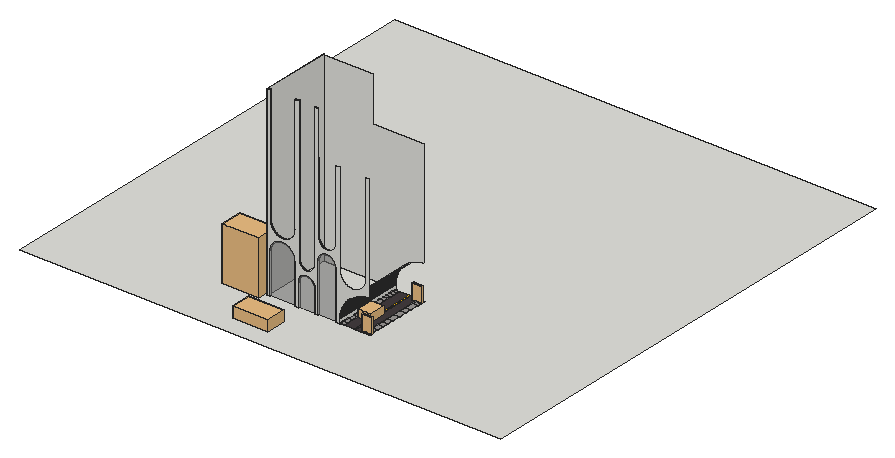
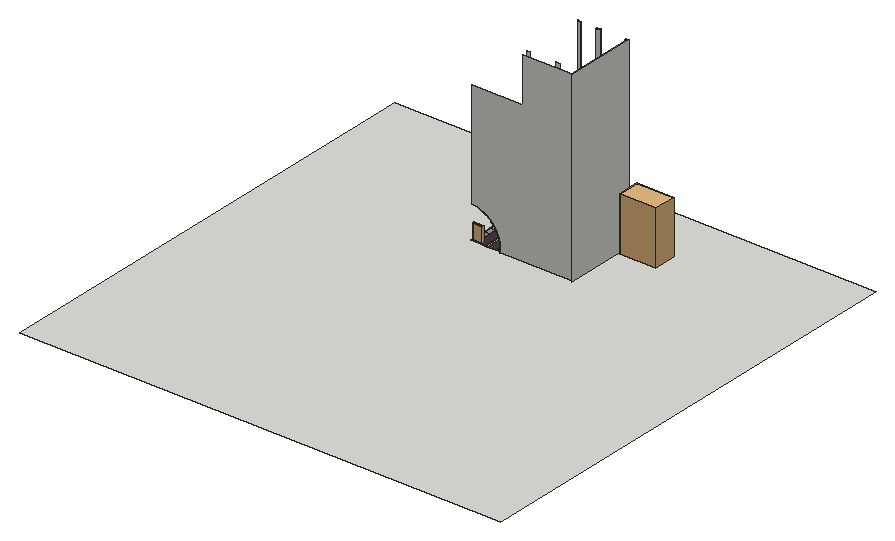
# SketchUp Ruby script. Lengths in inches.
U = 1.inch
M = Sketchup.active_model
def pt(a) = Geom::Point3d.new(a.map { |v| v * U })
def face(e, loops, mat)
  f = e.add_face(loops[0].map { |a| pt(a) })
  loops[1..].each { |l| e.add_face(l.map { |a| pt(a) }).erase! }
  f.material = f.back_material = mat if mat
  f
end
# faces: each face lists its corners as indices into pts; further lists are holes
def faces(e, pts, list, mat = nil) = list.each { |f| face(e, (f[0].is_a?(Array) ? f : [f]).map { |l| l.map { |i| pts[i] } }, mat) }
# xy, xz, yz: faces in a plane at the given z, y or x. An outline is a flat list of corners, or four numbers for a rectangle; further outlines are holes
def ring(l) = l.size == 4 ? [[l[0], l[1]], [l[2], l[1]], [l[2], l[3]], [l[0], l[3]]] : l.each_slice(2).to_a
def flat(e, list, mat, &to3) = list.each { |f| face(e, (f[0].is_a?(Array) ? f : [f]).map { |l| ring(l).map { |u, v| to3.(u, v) } }, mat) }
def xy(e, z, list, mat = nil) = flat(e, list, mat) { |x, y| [x, y, z] }
def xz(e, y, list, mat = nil) = flat(e, list, mat) { |x, z| [x, y, z] }
def yz(e, x, list, mat = nil) = flat(e, list, mat) { |y, z| [x, y, z] }
def lines(e, pts, list) = list.each { |a, b| e.add_line(pt(pts[a]), pt(pts[b])) }
# prism: a flat outline (further loops are holes) pulled along v
def prism(e, loops, v, mat = nil)
  f = face(e, loops, mat); d = Geom::Vector3d.new(v.map { |x| x * U })
  f.pushpull(f.normal.samedirection?(d) ? d.length : -d.length)
end
def box(e, o, s, mat = nil) = prism(e, [[o, [o[0] + s[0], o[1], o[2]], [o[0] + s[0], o[1] + s[1], o[2]], [o[0], o[1] + s[1], o[2]]]], [0, 0, s[2]], mat)
def at(x, y, z, deg = 0) = Geom::Transformation.translation(pt([x, y, z])) * Geom::Transformation.rotation(ORIGIN, Z_AXIS, deg.degrees)
def axes(o, x, y, z) = Geom::Transformation.new([*x, 0, *y, 0, *z, 0, *pt(o).to_a, 1])
def part(name) = M.definitions.add(name)
# library, detail: a bought-in or finely detailed component or shape, given as its bounding box
def library(name, o, s) = part(name).tap { |d| box(d.entities, o, s) }
def detail(e, o, s) = box(e.add_group.entities, o, s)
def put(e, d, t, mat = nil) = e.add_instance(d, t).tap { |i| i.material = mat if mat }
def group(e, t, mat = nil) = e.add_group.tap { |g| g.transformation = t; g.material = mat if mat }.entities
root = M.entities
M.materials.add("Asphalt_New").color = [67, 60, 62]
M.materials.add("Color_D01").color = [255, 191, 0]
M.materials.add("Concrete_Aggregate_Smoke").color = [154, 150, 148]
M.materials.add("[Translucent Glass Gray]").color = [128, 128, 128]
M.materials["[Translucent Glass Gray]"].alpha = 0.5
c1 = library("ske72",[-9.6875,-115.78,0],[19.375,125.47,218.23])
c2 = part("road")
xy(c2.entities,0,[[0,61.25,879,180.3125],[0,193.18,879,202.26],[0,211.38,879,312.5]],"Asphalt_New")
xy(c2.entities,0,[[0,180.3125,879,193.18],[0,202.26,879,211.38]],"Color_D01")
xy(c2.entities,2.25,[[0,0,58.96,61.25],[58.96,0,130.63,61.25],[130.63,0,205.31,61.25],[205.31,0,271.13,61.25],[271.13,0,347.96,61.25],
  [347.96,0,422.25,61.25],[422.25,0,490,61.25],[490,0,565.64,61.25],[565.64,0,642.8125,61.25],[642.8125,0,697.3125,61.25],
  [697.3125,0,742.61,61.25],[742.61,0,787.91,61.25],[787.91,0,833.2,61.25],[833.2,0,878.5,61.25],[0,312.5,55.73,383],
  [55.73,312.5,137.52,383],[137.52,312.5,221.8,383],[221.8,312.5,297.83,383],[297.83,312.5,375.9,383],[375.9,312.5,479.79,383],
  [479.79,312.5,571.31,383],[571.31,312.5,662.56,383],[662.56,312.5,768.4,383],[768.4,312.5,821.33,383],[821.33,312.5,874.25,383]],"Concrete_Aggregate_Smoke")
xz(c2.entities,0,[[0,0,58.96,2.25],[58.96,0,130.63,2.25],[130.63,0,205.31,2.25],[205.31,0,271.13,2.25],[271.13,0,347.96,2.25],
  [347.96,0,422.25,2.25],[422.25,0,490,2.25],[490,0,565.64,2.25],[565.64,0,604.23,2.25],[604.23,0,642.8125,2.25],
  [642.8125,0,697.3125,2.25],[697.3125,0,742.61,2.25],[742.61,0,787.91,2.25],[787.91,0,833.2,2.25],[833.2,0,878.5,2.25]],"Concrete_Aggregate_Smoke")
xz(c2.entities,61.25,[[0,0,58.96,2.25],[58.96,0,130.63,2.25],[130.63,0,205.31,2.25],[205.31,0,271.13,2.25],[271.13,0,347.96,2.25],
  [347.96,0,422.25,2.25],[422.25,0,490,2.25],[490,0,565.64,2.25],[565.64,0,642.8125,2.25],[642.8125,0,697.3125,2.25],
  [697.3125,0,742.61,2.25],[742.61,0,787.91,2.25],[787.91,0,833.2,2.25],[833.2,0,878.5,2.25]],"Concrete_Aggregate_Smoke")
xz(c2.entities,312.5,[[0,0,55.73,2.25],[55.73,0,137.52,2.25],[137.52,0,221.8,2.25],[221.8,0,297.83,2.25],[297.83,0,373.56,2.25],
  [373.56,0,375.9,2.25],[375.9,0,479.79,2.25],[479.79,0,571.31,2.25],[571.31,0,662.56,2.25],[662.56,0,768.4,2.25],
  [768.4,0,821.33,2.25],[821.33,0,874.25,2.25]],"Concrete_Aggregate_Smoke")
xz(c2.entities,383,[[0,0,55.73,2.25],[55.73,0,137.52,2.25],[137.52,0,221.8,2.25],[221.8,0,297.83,2.25],[297.83,0,375.9,2.25],
  [375.9,0,479.79,2.25],[479.79,0,571.31,2.25],[571.31,0,662.56,2.25],[662.56,0,768.4,2.25],[768.4,0,821.33,2.25],
  [821.33,0,874.25,2.25]],"Concrete_Aggregate_Smoke")
yz(c2.entities,0,[[0,0,61.25,2.25],[312.5,0,383,2.25]],"Concrete_Aggregate_Smoke")
yz(c2.entities,874.25,[[312.5,0,383,2.25]],"Concrete_Aggregate_Smoke")
yz(c2.entities,878.5,[[0,0,61.25,2.25]],"Concrete_Aggregate_Smoke")
p = [[0,0,0],[-0.25,0,0]]
lines(c2.entities,p,[[0,1]])
put(c2.entities,c1,at(36.91,376.45,-15.96))
put(c2.entities,c1,at(842.66,376.45,-15.96))
c3 = library("2016+Honda+Civic+LX+Sedan",[0.01,0.03,0.02],[16.17,34.46,10.62])
c4 = library("006_cordyline_australis",[-46.19,-61.57,-0.26],[141.35,155.27,163.93])
c5 = library("car",[-0.875,0,0],[16.18,34.45,10.62])
xy(root,0,[[0,0,3621,3534]])
xz(root,487.08,[[1470.625,0,1494.625,0,1494.625,300.79,1494.8125,306.78,1495.375,312.74,1496.3125,318.66,1497.62,324.51,1499.29,330.27,1501.32,335.9,1503.7,341.4,1506.42,346.74,1509.47,351.9,1512.84,356.86,1516.52,361.59,1520.48,366.09,1524.72,370.33,1529.21,374.29,1533.95,377.96,1538.9,381.33,1544.0625,384.38,1549.4,387.1,1554.9,389.48,1560.54,391.51,1566.3,393.1875,1572.14,394.49,1578.0625,395.43,1584.03,395.99,1590.02,396.18,1596.01,395.99,1601.98,395.43,1607.9,394.49,1613.74,393.1875,1619.5,391.51,1625.14,389.48,1630.64,387.1,1635.98,384.38,1641.14,381.33,1646.09,377.96,1650.83,374.29,1655.32,370.33,1659.5625,366.09,1663.52,361.59,1667.2,356.86,1670.57,351.9,1673.62,346.74,1676.34,341.4,1678.72,335.9,1680.75,330.27,1682.42,324.51,1683.73,318.66,1684.66,312.74,1685.23,306.78,1685.42,300.79,1685.42,0,1709.42,0,1709.42,171.3125,1709.54,175.19,1709.9,179.04,1710.51,182.87,1711.35,186.65,1712.43,190.37,1713.75,194.01,1715.28,197.5625,1717.04,201.01,1719.01,204.35,1721.19,207.55,1723.5625,210.61,1726.125,213.52,1728.86,216.26,1731.77,218.82,1734.83,221.19,1738.03,223.37,1741.37,225.34,1744.82,227.1,1748.37,228.63,1752.02,229.95,1755.73,231.03,1759.51,231.87,1763.34,232.48,1767.2,232.84,1771.07,232.96,1774.9375,232.84,1778.79,232.48,1782.62,231.87,1786.4,231.03,1790.12,229.95,1793.76,228.63,1797.32,227.1,1800.77,225.34,1804.1,223.37,1807.3,221.19,1810.36,218.82,1813.27,216.26,1816.01,213.52,1818.57,210.61,1820.94,207.55,1823.12,204.35,1825.09,201.01,1826.85,197.5625,1828.39,194.01,1829.7,190.37,1830.78,186.65,1831.625,182.87,1832.23,179.04,1832.59,175.19,1832.72,171.3125,1832.72,0,1856.72,0,1856.72,362.73,1856.85,366.99,1857.25,371.24,1857.92,375.46,1858.85,379.62,1860.04,383.72,1861.49,387.74,1863.18,391.65,1865.12,395.45,1867.29,399.13,1869.6875,402.66,1872.3,406.03,1875.125,409.23,1878.14,412.25,1881.35,415.07,1884.72,417.68,1888.25,420.08,1891.92,422.26,1895.72,424.19,1899.64,425.89,1903.65,427.33,1907.75,428.52,1911.92,429.45,1916.13,430.12,1920.38,430.52,1924.64,430.66,1928.91,430.52,1933.16,430.12,1937.37,429.45,1941.54,428.52,1945.64,427.33,1949.65,425.89,1953.57,424.19,1957.125,422.38,1957.37,422.26,1961.04,420.08,1964.57,417.68,1967.94,415.07,1971.14,412.25,1974.16,409.23,1976.98,406.03,1979.6,402.66,1982,399.13,1984.17,395.45,1986.11,391.65,1987.8,387.74,1989.25,383.72,1990.4375,379.62,1991.37,375.46,1992.04,371.24,1992.4375,366.99,1992.57,362.73,1992.57,0,2019.16,0,2018.78,7.52,2018.64,15.05,2018.74,22.58,2019.07,30.1,2019.16,31.18,2019.64,37.6,2020.44,45.09,2021.48,52.55,2022.75,59.97,2024.25,67.35,2025.98,74.67,2027.94,81.94,2030.13,89.15,2032.54,96.28,2035.17,103.33,2038.02,110.3,2041.09,117.18,2044.375,123.95,2047.87,130.62,2051.57,137.18,2055.47,143.62,2059.57,149.93,2063.875,156.11,2068.36,162.15,2073.04,168.05,2077.9,173.8,2082.94,179.4,2088.14,184.84,2093.52,190.11,2099.06,195.21,2104.76,200.13,2110.6,204.87,2116.6,209.43,2122.73,213.8,2129,217.97,2135.39,221.95,2141.9,225.72,2148.53,229.29,2155.27,232.64,2162.11,235.79,2169.05,238.72,2176.07,241.43,2183.18,243.92,2190.36,246.19,2197.6,248.23,2204.91,250.04,2212.27,251.63,2218.1,252.69,2219.68,252.98,2227.12,254.1,2233.1,254.8125,2234.6,254.99,2242.1,255.64,2242.1,1054,2218.1,1054,2218.1,364.18,2217.9,357.93,2217.3125,351.71,2216.34,345.54,2214.97,339.4375,2213.23,333.4375,2211.11,327.56,2208.63,321.82,2205.79,316.26,2202.61,310.88,2199.1,305.71,2195.27,300.77,2191.14,296.08,2186.72,291.67,2182.03,287.53,2177.09,283.7,2171.93,280.19,2166.55,277.01,2160.98,274.17,2155.24,271.69,2149.37,269.57,2143.36,267.83,2137.27,266.47,2131.09,265.49,2124.87,264.9,2118.63,264.71,2112.38,264.9,2106.16,265.49,2099.99,266.47,2093.89,267.83,2087.89,269.57,2082.01,271.69,2076.27,274.17,2070.71,277.01,2065.33,280.19,2060.16,283.7,2055.22,287.53,2050.53,291.67,2046.12,296.08,2041.98,300.77,2038.15,305.71,2034.64,310.88,2031.46,316.26,2028.62,321.82,2026.14,327.56,2024.02,333.4375,2022.28,339.4375,2020.92,345.54,2019.94,351.71,2019.35,357.93,2019.16,364.18,2019.16,1054,1992.57,1054,1992.57,527,1992.4375,522.73,1992.04,518.49,1991.37,514.27,1990.4375,510.11,1989.25,506.01,1987.8,501.99,1986.11,498.08,1984.17,494.28,1982,490.6,1979.6,487.07,1976.98,483.7,1974.16,480.5,1971.14,477.48,1967.94,474.66,1964.57,472.04,1961.04,469.65,1957.37,467.47,1953.57,465.54,1949.65,463.84,1945.64,462.4,1941.54,461.21,1937.37,460.27,1933.16,459.61,1928.91,459.21,1924.64,459.07,1920.38,459.21,1916.13,459.61,1911.92,460.27,1907.75,461.21,1903.65,462.4,1899.64,463.84,1895.72,465.54,1891.92,467.47,1888.25,469.65,1884.72,472.04,1881.35,474.66,1878.14,477.48,1875.125,480.5,1872.3,483.7,1869.6875,487.07,1867.29,490.6,1865.12,494.28,1863.18,498.08,1861.49,501.99,1860.04,506.01,1858.85,510.11,1857.92,514.27,1857.25,518.49,1856.85,522.73,1856.72,527,1856.72,1394,1832.72,1394,1832.72,325.5,1832.59,321.63,1832.23,317.77,1831.625,313.95,1830.78,310.17,1829.7,306.45,1828.39,302.8,1826.85,299.25,1825.09,295.8,1823.12,292.47,1820.94,289.26,1818.57,286.2,1816.01,283.3,1813.27,280.56,1810.36,278,1807.3,275.625,1804.1,273.45,1800.77,271.48,1797.32,269.72,1793.76,268.18,1790.12,266.87,1786.4,265.79,1782.62,264.94,1778.79,264.34,1774.9375,263.97,1771.07,263.85,1767.2,263.97,1763.34,264.34,1759.51,264.94,1755.73,265.79,1752.02,266.87,1748.37,268.18,1744.82,269.72,1741.37,271.48,1738.03,273.45,1734.83,275.625,1731.77,278,1728.86,280.56,1726.125,283.3,1723.5625,286.2,1721.19,289.26,1719.01,292.47,1717.04,295.8,1715.28,299.25,1713.75,302.8,1712.43,306.45,1711.35,310.17,1710.51,313.95,1709.9,317.77,1709.54,321.63,1709.42,325.5,1709.42,1394,1685.42,1394,1685.42,523.51,1685.82,517.14,1685.79,510.75,1685.42,505.5,1685.34,504.38,1684.46,498.05,1683.17,491.8,1681.46,485.64,1679.34,479.62,1676.83,473.74,1673.93,468.05,1670.66,462.5625,1667.03,457.31,1663.0625,452.3,1658.77,447.57,1654.17,443.14,1649.28,439.03,1644.13,435.25,1638.74,431.82,1633.14,428.76,1627.34,426.07,1621.375,423.78,1615.27,421.9,1609.06,420.42,1602.76,419.36,1596.4,418.72,1590.02,418.51,1583.64,418.72,1577.28,419.36,1570.98,420.42,1564.77,421.9,1558.66,423.78,1552.7,426.07,1546.9,428.76,1541.3,431.82,1535.91,435.25,1530.76,439.03,1525.875,443.14,1521.27,447.57,1516.98,452.3,1513.01,457.31,1509.38,462.5625,1506.11,468.05,1503.21,473.74,1500.7,479.62,1498.58,485.64,1496.875,491.8,1495.58,498.05,1494.7,504.38,1494.625,505.5,1494.25,510.75,1494.22,517.14,1494.625,523.51,1494.625,1394,1470.625,1394],[2019.16,0,2019.16,31.18,2019.07,30.1,2018.74,22.58,2018.64,15.05,2018.78,7.52]])
xz(root,487.08,[[1494.625,0,1685.42,0,1685.42,300.79,1685.23,306.78,1684.66,312.74,1683.73,318.66,1682.42,324.51,1680.75,330.27,1678.72,335.9,1676.34,341.4,1673.62,346.74,1670.57,351.9,1667.2,356.86,1663.52,361.59,1659.5625,366.09,1655.32,370.33,1650.83,374.29,1646.09,377.96,1641.14,381.33,1635.98,384.38,1630.64,387.1,1625.14,389.48,1619.5,391.51,1613.74,393.1875,1607.9,394.49,1601.98,395.43,1596.01,395.99,1590.02,396.18,1584.03,395.99,1578.0625,395.43,1572.14,394.49,1566.3,393.1875,1560.54,391.51,1554.9,389.48,1549.4,387.1,1544.0625,384.38,1538.9,381.33,1533.95,377.96,1529.21,374.29,1524.72,370.33,1520.48,366.09,1516.52,361.59,1512.84,356.86,1509.47,351.9,1506.42,346.74,1503.7,341.4,1501.32,335.9,1499.29,330.27,1497.62,324.51,1496.3125,318.66,1495.375,312.74,1494.8125,306.78,1494.625,300.79],[1709.42,0,1832.72,0,1832.72,171.3125,1832.59,175.19,1832.23,179.04,1831.625,182.87,1830.78,186.65,1829.7,190.37,1828.39,194.01,1826.85,197.5625,1825.09,201.01,1823.12,204.35,1820.94,207.55,1818.57,210.61,1816.01,213.52,1813.27,216.26,1810.36,218.82,1807.3,221.19,1804.1,223.37,1800.77,225.34,1797.32,227.1,1793.76,228.63,1790.12,229.95,1786.4,231.03,1782.62,231.87,1778.79,232.48,1774.9375,232.84,1771.07,232.96,1767.2,232.84,1763.34,232.48,1759.51,231.87,1755.73,231.03,1752.02,229.95,1748.37,228.63,1744.82,227.1,1741.37,225.34,1738.03,223.37,1734.83,221.19,1731.77,218.82,1728.86,216.26,1726.125,213.52,1723.5625,210.61,1721.19,207.55,1719.01,204.35,1717.04,201.01,1715.28,197.5625,1713.75,194.01,1712.43,190.37,1711.35,186.65,1710.51,182.87,1709.9,179.04,1709.54,175.19,1709.42,171.3125],[1856.72,0,1992.57,0,1992.57,362.73,1992.4375,366.99,1992.04,371.24,1991.37,375.46,1990.4375,379.62,1989.25,383.72,1987.8,387.74,1986.11,391.65,1984.17,395.45,1982,399.13,1979.6,402.66,1976.98,406.03,1974.16,409.23,1971.14,412.25,1967.94,415.07,1964.57,417.68,1961.04,420.08,1957.37,422.26,1953.57,424.19,1949.65,425.89,1945.64,427.33,1941.54,428.52,1937.37,429.45,1933.16,430.12,1928.91,430.52,1924.64,430.66,1920.38,430.52,1916.13,430.12,1911.92,429.45,1907.75,428.52,1903.65,427.33,1899.64,425.89,1895.72,424.19,1891.92,422.26,1888.25,420.08,1884.72,417.68,1881.35,415.07,1878.14,412.25,1875.125,409.23,1872.3,406.03,1869.6875,402.66,1867.29,399.13,1865.12,395.45,1863.18,391.65,1861.49,387.74,1860.04,383.72,1858.85,379.62,1857.92,375.46,1857.25,371.24,1856.85,366.99,1856.72,362.73]],"[Translucent Glass Gray]")
xz(root,496.08,[[1479.625,0,1479.625,1394,1494.625,1394,1494.625,505.5,1494.7,504.38,1495.58,498.05,1496.875,491.8,1498.58,485.64,1500.7,479.62,1503.21,473.74,1506.11,468.05,1509.38,462.5625,1513.01,457.31,1516.98,452.3,1521.27,447.57,1525.875,443.14,1530.76,439.03,1535.91,435.25,1541.3,431.82,1546.9,428.76,1552.7,426.07,1558.66,423.78,1564.77,421.9,1570.98,420.42,1577.28,419.36,1583.64,418.72,1590.02,418.51,1596.4,418.72,1602.76,419.36,1609.06,420.42,1615.27,421.9,1621.375,423.78,1627.34,426.07,1633.14,428.76,1638.74,431.82,1644.13,435.25,1649.28,439.03,1654.17,443.14,1658.77,447.57,1663.0625,452.3,1667.03,457.31,1670.66,462.5625,1673.93,468.05,1676.83,473.74,1679.34,479.62,1681.46,485.64,1683.17,491.8,1684.46,498.05,1685.34,504.38,1685.42,505.5,1685.42,1394,1709.42,1394,1709.42,325.5,1709.54,321.63,1709.9,317.77,1710.51,313.95,1711.35,310.17,1712.43,306.45,1713.75,302.8,1715.28,299.25,1717.04,295.8,1719.01,292.47,1721.19,289.26,1723.5625,286.2,1726.125,283.3,1728.86,280.56,1731.77,278,1734.83,275.625,1738.03,273.45,1741.37,271.48,1744.82,269.72,1748.37,268.18,1752.02,266.87,1755.73,265.79,1759.51,264.94,1763.34,264.34,1767.2,263.97,1771.07,263.85,1774.9375,263.97,1778.79,264.34,1782.62,264.94,1786.4,265.79,1790.12,266.87,1793.76,268.18,1797.32,269.72,1800.77,271.48,1804.1,273.45,1807.3,275.625,1810.36,278,1813.27,280.56,1816.01,283.3,1818.57,286.2,1820.94,289.26,1823.12,292.47,1825.09,295.8,1826.85,299.25,1828.39,302.8,1829.7,306.45,1830.78,310.17,1831.625,313.95,1832.23,317.77,1832.59,321.63,1832.72,325.5,1832.72,1394,1847.72,1394,1847.72,1054,1856.72,1054,1856.72,527,1856.85,522.73,1857.25,518.49,1857.92,514.27,1858.85,510.11,1860.04,506.01,1861.49,501.99,1863.18,498.08,1865.12,494.28,1867.29,490.6,1869.6875,487.07,1872.3,483.7,1875.125,480.5,1878.14,477.48,1881.35,474.66,1884.72,472.04,1888.25,469.65,1891.92,467.47,1895.72,465.54,1899.64,463.84,1903.65,462.4,1907.75,461.21,1911.92,460.27,1916.13,459.61,1920.38,459.21,1924.64,459.07,1928.91,459.21,1933.16,459.61,1937.37,460.27,1941.54,461.21,1945.64,462.4,1949.65,463.84,1953.57,465.54,1957.125,467.35,1957.125,422.38,1953.57,424.19,1949.65,425.89,1945.64,427.33,1941.54,428.52,1937.37,429.45,1933.16,430.12,1928.91,430.52,1924.64,430.66,1920.38,430.52,1916.13,430.12,1911.92,429.45,1907.75,428.52,1903.65,427.33,1899.64,425.89,1895.72,424.19,1891.92,422.26,1888.25,420.08,1884.72,417.68,1881.35,415.07,1878.14,412.25,1875.125,409.23,1872.3,406.03,1869.6875,402.66,1867.29,399.13,1865.12,395.45,1863.18,391.65,1861.49,387.74,1860.04,383.72,1858.85,379.62,1857.92,375.46,1857.25,371.24,1856.85,366.99,1856.72,362.73,1856.72,0,1832.72,0,1832.72,171.3125,1832.59,175.19,1832.23,179.04,1831.625,182.87,1830.78,186.65,1829.7,190.37,1828.39,194.01,1826.85,197.5625,1825.09,201.01,1823.12,204.35,1820.94,207.55,1818.57,210.61,1816.01,213.52,1813.27,216.26,1810.36,218.82,1807.3,221.19,1804.1,223.37,1800.77,225.34,1797.32,227.1,1793.76,228.63,1790.12,229.95,1786.4,231.03,1782.62,231.87,1778.79,232.48,1774.9375,232.84,1771.07,232.96,1767.2,232.84,1763.34,232.48,1759.51,231.87,1755.73,231.03,1752.02,229.95,1748.37,228.63,1744.82,227.1,1741.37,225.34,1738.03,223.37,1734.83,221.19,1731.77,218.82,1728.86,216.26,1726.125,213.52,1723.5625,210.61,1721.19,207.55,1719.01,204.35,1717.04,201.01,1715.28,197.5625,1713.75,194.01,1712.43,190.37,1711.35,186.65,1710.51,182.87,1709.9,179.04,1709.54,175.19,1709.42,171.3125,1709.42,0,1685.42,0,1685.42,300.79,1685.23,306.78,1684.66,312.74,1683.73,318.66,1682.42,324.51,1680.75,330.27,1678.72,335.9,1676.34,341.4,1673.62,346.74,1670.57,351.9,1667.2,356.86,1663.52,361.59,1659.5625,366.09,1655.32,370.33,1650.83,374.29,1646.09,377.96,1641.14,381.33,1635.98,384.38,1630.64,387.1,1625.14,389.48,1619.5,391.51,1613.74,393.1875,1607.9,394.49,1601.98,395.43,1596.01,395.99,1590.02,396.18,1584.03,395.99,1578.0625,395.43,1572.14,394.49,1566.3,393.1875,1560.54,391.51,1554.9,389.48,1549.4,387.1,1544.0625,384.38,1538.9,381.33,1533.95,377.96,1529.21,374.29,1524.72,370.33,1520.48,366.09,1516.52,361.59,1512.84,356.86,1509.47,351.9,1506.42,346.74,1503.7,341.4,1501.32,335.9,1499.29,330.27,1497.62,324.51,1496.3125,318.66,1495.375,312.74,1494.8125,306.78,1494.625,300.79,1494.625,0]])
xz(root,1012.08,[[1479.625,0,2019.16,0,2019.16,31.18,2019.64,37.6,2020.44,45.09,2021.48,52.55,2022.75,59.97,2024.25,67.35,2025.98,74.67,2027.94,81.94,2030.13,89.15,2032.54,96.28,2035.17,103.33,2038.02,110.3,2041.09,117.18,2044.375,123.95,2047.87,130.62,2051.57,137.18,2055.47,143.62,2059.57,149.93,2063.875,156.11,2068.36,162.15,2073.04,168.05,2077.9,173.8,2082.94,179.4,2088.14,184.84,2093.52,190.11,2099.06,195.21,2104.76,200.13,2110.6,204.87,2116.6,209.43,2122.73,213.8,2129,217.97,2135.39,221.95,2141.9,225.72,2148.53,229.29,2155.27,232.64,2162.11,235.79,2169.05,238.72,2176.07,241.43,2183.18,243.92,2190.36,246.19,2197.6,248.23,2204.91,250.04,2212.27,251.63,2218.1,252.69,2219.68,252.98,2227.12,254.1,2233.1,254.8125,2233.1,1054,1847.72,1054,1847.72,1394,1479.625,1394]])
yz(root,1470.625,[[487.08,0,1021.08,1394]])
yz(root,1479.625,[[496.08,0,1012.08,1394]])
yz(root,1494.625,[[487.08,0,496.08,300.79]])
yz(root,1685.42,[[487.08,0,496.08,300.79]])
yz(root,1709.42,[[487.08,0,496.08,171.3125]])
yz(root,1832.72,[[487.08,0,496.08,171.3125]])
yz(root,1856.72,[[487.08,0,496.08,362.73]])
yz(root,1992.57,[[487.08,0,496.08,362.73]])
yz(root,2019.16,[[487.08,0,1012.08,31.18]])
p = [[2019.64,487.08,37.6],[2019.16,487.08,31.18],[2019.16,1012.08,31.18],[2019.64,1012.08,37.6],[2020.44,1012.08,45.09],[2020.44,487.08,45.09],
  [2021.48,487.08,52.55],[2021.48,1012.08,52.55],[2022.75,487.08,59.97],[2022.75,1012.08,59.97],[2024.25,487.08,67.35],[2024.25,1012.08,67.35],
  [2025.98,487.08,74.67],[2025.98,1012.08,74.67],[2027.94,487.08,81.94],[2027.94,1012.08,81.94],[2030.13,487.08,89.15],[2030.13,1012.08,89.15],
  [2032.54,1012.08,96.28],[2032.54,487.08,96.28],[2035.17,487.08,103.33],[2035.17,1012.08,103.33],[2038.02,487.08,110.3],[2038.02,1012.08,110.3],
  [2041.09,487.08,117.18],[2041.09,1012.08,117.18],[2044.375,487.08,123.95],[2044.375,1012.08,123.95],[2047.87,487.08,130.62],[2047.87,1012.08,130.62],
  [2051.57,487.08,137.18],[2051.57,1012.08,137.18],[2055.47,487.08,143.62],[2055.47,1012.08,143.62],[2059.57,487.08,149.93],[2059.57,1012.08,149.93],
  [2063.875,487.08,156.11],[2063.875,1012.08,156.11],[2068.36,487.08,162.15],[2068.36,1012.08,162.15],[2073.04,487.08,168.05],[2073.04,1012.08,168.05],
  [2077.9,487.08,173.8],[2077.9,1012.08,173.8],[1709.54,487.08,175.19],[1709.42,487.08,171.3125],[1709.42,496.08,171.3125],[1709.54,496.08,175.19],
  [1832.72,487.08,171.3125],[1832.59,487.08,175.19],[1832.59,496.08,175.19],[1832.72,496.08,171.3125],[2082.94,487.08,179.4],[2082.94,1012.08,179.4],
  [1709.9,487.08,179.04],[1709.9,496.08,179.04],[1832.23,487.08,179.04],[1832.23,496.08,179.04],[1710.51,487.08,182.87],[1710.51,496.08,182.87],
  [1831.625,487.08,182.87],[1831.625,496.08,182.87],[2088.14,487.08,184.84],[2088.14,1012.08,184.84],[1711.35,487.08,186.65],[1711.35,496.08,186.65],
  [1830.78,487.08,186.65],[1830.78,496.08,186.65],[2093.52,487.08,190.11],[2093.52,1012.08,190.11],[1712.43,487.08,190.37],[1712.43,496.08,190.37],
  [1829.7,487.08,190.37],[1829.7,496.08,190.37],[2099.06,487.08,195.21],[2099.06,1012.08,195.21],[1713.75,487.08,194.01],[1713.75,496.08,194.01],
  [1828.39,487.08,194.01],[1828.39,496.08,194.01],[1715.28,487.08,197.5625],[1715.28,496.08,197.5625],[1826.85,487.08,197.5625],[1826.85,496.08,197.5625],
  [2104.76,487.08,200.13],[2104.76,1012.08,200.13],[1717.04,487.08,201.01],[1717.04,496.08,201.01],[1825.09,487.08,201.01],[1825.09,496.08,201.01],
  [2110.6,487.08,204.87],[2110.6,1012.08,204.87],[1719.01,487.08,204.35],[1719.01,496.08,204.35],[1823.12,487.08,204.35],[1823.12,496.08,204.35],
  [1721.19,487.08,207.55],[1721.19,496.08,207.55],[1820.94,487.08,207.55],[1820.94,496.08,207.55],[2116.6,487.08,209.43],[2116.6,1012.08,209.43],
  [1723.5625,487.08,210.61],[1723.5625,496.08,210.61],[1818.57,487.08,210.61],[1818.57,496.08,210.61],[2122.73,487.08,213.8],[2122.73,1012.08,213.8],
  [1726.125,487.08,213.52],[1726.125,496.08,213.52],[1816.01,487.08,213.52],[1816.01,496.08,213.52],[1728.86,487.08,216.26],[1728.86,496.08,216.26],
  [1813.27,487.08,216.26],[1813.27,496.08,216.26],[2129,487.08,217.97],[2129,1012.08,217.97],[1731.77,487.08,218.82],[1731.77,496.08,218.82],
  [1810.36,487.08,218.82],[1810.36,496.08,218.82],[2135.39,487.08,221.95],[2135.39,1012.08,221.95],[1734.83,487.08,221.19],[1734.83,496.08,221.19],
  [1807.3,487.08,221.19],[1807.3,496.08,221.19],[1738.03,487.08,223.37],[1738.03,496.08,223.37],[1804.1,487.08,223.37],[1804.1,496.08,223.37],
  [2141.9,487.08,225.72],[2141.9,1012.08,225.72],[1741.37,487.08,225.34],[1741.37,496.08,225.34],[1800.77,487.08,225.34],[1800.77,496.08,225.34],
  [1744.82,487.08,227.1],[1744.82,496.08,227.1],[1797.32,487.08,227.1],[1797.32,496.08,227.1],[2148.53,487.08,229.29],[2148.53,1012.08,229.29],
  [1992.57,496.08,0],[2019.16,496.08,0]]
faces(root,p,[[0,1,2,3],[4,5,0,3],[6,5,4,7],[8,6,7,9],[10,8,9,11],[12,10,11,13],[14,12,13,15],[16,14,15,17],
  [18,19,16,17],[20,19,18,21],[22,20,21,23],[24,22,23,25],[26,24,25,27],[28,26,27,29],[30,28,29,31],[32,30,31,33],
  [34,32,33,35],[36,34,35,37],[38,36,37,39],[40,38,39,41],[42,40,41,43],[44,45,46,47],[48,49,50,51],[52,42,43,53],
  [54,44,47,55],[49,56,57,50],[58,54,55,59],[56,60,61,57],[62,52,53,63],[64,58,59,65],[60,66,67,61],[68,62,63,69],
  [70,64,65,71],[66,72,73,67],[74,68,69,75],[76,70,71,77],[72,78,79,73],[80,76,77,81],[78,82,83,79],[84,74,75,85],
  [86,80,81,87],[82,88,89,83],[90,84,85,91],[92,86,87,93],[88,94,95,89],[96,92,93,97],[94,98,99,95],[100,90,91,101],
  [102,96,97,103],[98,104,105,99],[106,100,101,107],[108,102,103,109],[104,110,111,105],[112,108,109,113],[110,114,115,111],[116,106,107,117],
  [118,112,113,119],[114,120,121,115],[122,116,117,123],[124,118,119,125],[120,126,127,121],[128,124,125,129],[126,130,131,127],[132,122,123,133],
  [134,128,129,135],[130,136,137,131],[138,134,135,139],[136,140,141,137],[142,132,133,143]])
lines(root,p,[[144,145]])
put(root,c2,axes([2019.16,487.23,0.5],[0,0.59,0],[0.59,0,0],[0,0,0.5478]))
put(root,c3,axes([1750.05,145.2,-0.17],[0,9.24,0],[-7.6551,0,0],[0,0,7.7153]))
put(root,c4,axes([1368.03,492.48,5.26],[-1.93979,0,0],[0,1.06864,0],[0,0,2.45283]))
put(root,c5,axes([2082.54,584.99,20],[6.1908,0,0],[0,3.5979,0],[0,0,5.55502]))
